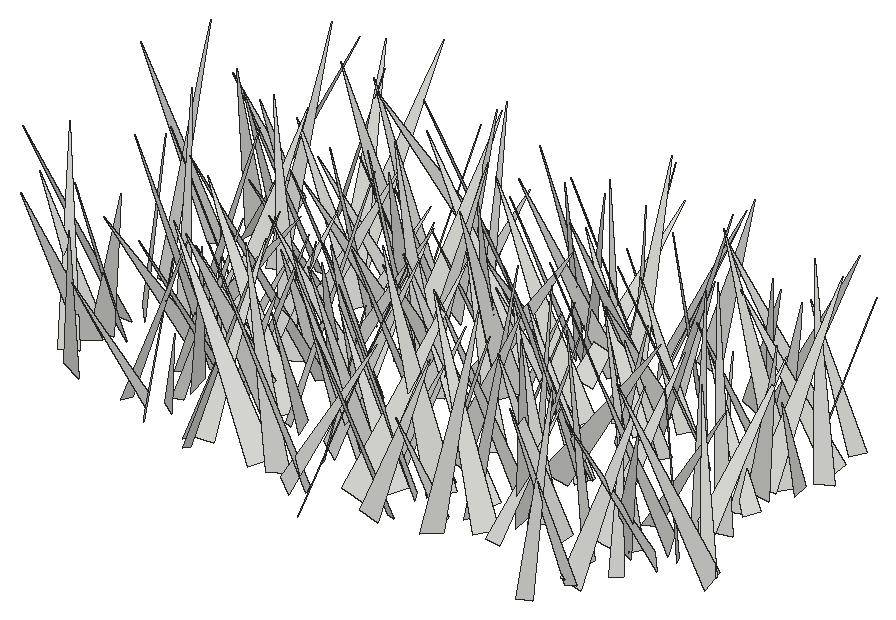
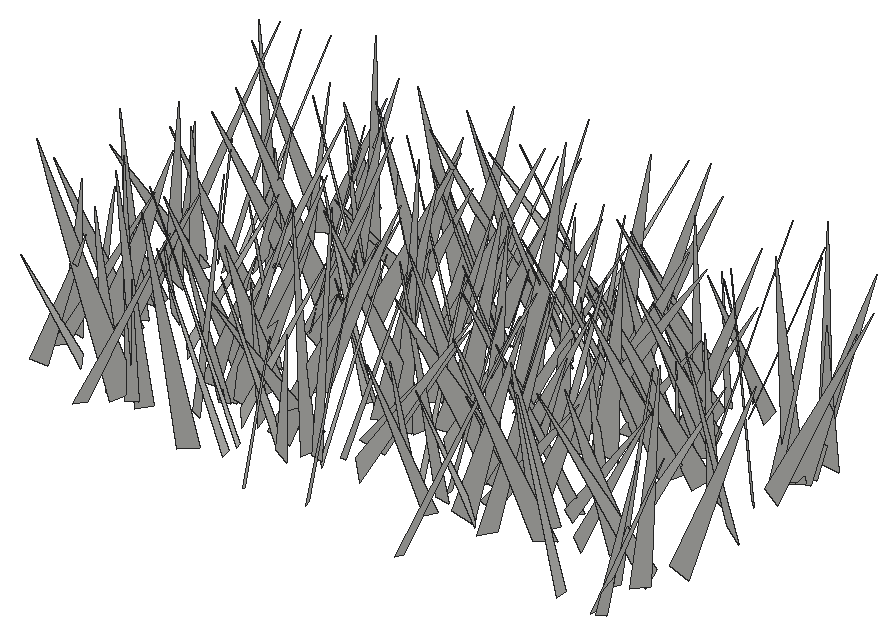
# SketchUp Ruby script. Lengths in inches.
U = 1.inch
M = Sketchup.active_model
def pt(a) = Geom::Point3d.new(a.map { |v| v * U })
def face(e, loops, mat)
  f = e.add_face(loops[0].map { |a| pt(a) })
  loops[1..].each { |l| e.add_face(l.map { |a| pt(a) }).erase! }
  f.material = f.back_material = mat if mat
  f
end
# faces: each face lists its corners as indices into pts; further lists are holes
def faces(e, pts, list, mat = nil) = list.each { |f| face(e, (f[0].is_a?(Array) ? f : [f]).map { |l| l.map { |i| pts[i] } }, mat) }
# xy, xz, yz: faces in a plane at the given z, y or x. An outline is a flat list of corners, or four numbers for a rectangle; further outlines are holes
def ring(l) = l.size == 4 ? [[l[0], l[1]], [l[2], l[1]], [l[2], l[3]], [l[0], l[3]]] : l.each_slice(2).to_a
def flat(e, list, mat, &to3) = list.each { |f| face(e, (f[0].is_a?(Array) ? f : [f]).map { |l| ring(l).map { |u, v| to3.(u, v) } }, mat) }
def xy(e, z, list, mat = nil) = flat(e, list, mat) { |x, y| [x, y, z] }
def xz(e, y, list, mat = nil) = flat(e, list, mat) { |x, z| [x, y, z] }
def yz(e, x, list, mat = nil) = flat(e, list, mat) { |y, z| [x, y, z] }
def lines(e, pts, list) = list.each { |a, b| e.add_line(pt(pts[a]), pt(pts[b])) }
# prism: a flat outline (further loops are holes) pulled along v
def prism(e, loops, v, mat = nil)
  f = face(e, loops, mat); d = Geom::Vector3d.new(v.map { |x| x * U })
  f.pushpull(f.normal.samedirection?(d) ? d.length : -d.length)
end
def box(e, o, s, mat = nil) = prism(e, [[o, [o[0] + s[0], o[1], o[2]], [o[0] + s[0], o[1] + s[1], o[2]], [o[0], o[1] + s[1], o[2]]]], [0, 0, s[2]], mat)
def at(x, y, z, deg = 0) = Geom::Transformation.translation(pt([x, y, z])) * Geom::Transformation.rotation(ORIGIN, Z_AXIS, deg.degrees)
def axes(o, x, y, z) = Geom::Transformation.new([*x, 0, *y, 0, *z, 0, *pt(o).to_a, 1])
def part(name) = M.definitions.add(name)
# library, detail: a bought-in or finely detailed component or shape, given as its bounding box
def library(name, o, s) = part(name).tap { |d| box(d.entities, o, s) }
def detail(e, o, s) = box(e.add_group.entities, o, s)
def put(e, d, t, mat = nil) = e.add_instance(d, t).tap { |i| i.material = mat if mat }
def group(e, t, mat = nil) = e.add_group.tap { |g| g.transformation = t; g.material = mat if mat }.entities
root = M.entities
c1 = part("fur_instance\#9")
p = [[0.8125,0,1.79],[0.67,-0.02,1.48],[0,-0.11,0],[0,0.11,0]]
faces(c1.entities,p,[[0,1,2,3]])
put(root,c1,axes([463.09,264.2,-21.66],[-4.74866,-3.13825,0.27488],[-2.86364,4.50737,1.98925],[1.31291,-1.51952,5.33303]))
put(root,c1,axes([483.28,262.19,-21.66],[-3.66042,-4.84933,0.70173],[-4.78346,3.34689,-1.82316],[-1.06154,1.63996,5.79575]))
put(root,c1,axes([482.21,261.42,-21.66],[1.25839,-5.65908,2.69216],[-6.0262,-0.33916,2.10388],[1.71982,2.95233,5.40207]))
put(root,c1,axes([477.375,261.69,-21.66],[-7.14593,-4.06809,0.00282],[-3.91681,6.87864,-2.22635],[-1.09909,1.93614,7.91562]))
put(root,c1,axes([476.01,261.17,-21.66],[3.46284,5.45761,0.55951],[5.19477,-3.049,-2.40992],[1.76435,-1.73432,5.99742]))
put(root,c1,axes([457.36,264.17,-21.66],[-1.15928,-6.64992,1.1524],[-6.36185,1.46707,2.06591],[2.25307,0.72087,6.42631]))
put(root,c1,axes([486.22,263.67,-21.66],[-4.22859,-0.79072,0.99748],[-0.41595,4.12901,1.5098],[1.20299,-1.35177,4.02824]))
put(root,c1,axes([495.81,259.29,-21.66],[-6.32088,1.55628,0.92222],[1.03646,5.86264,-2.78949],[1.48264,2.53644,5.88169]))
put(root,c1,axes([496.86,262.39,-21.66],[-1.92463,-5.23066,1.71698],[-5.26178,1.21283,-2.20335],[-1.6191,2.27625,5.1195]))
put(root,c1,axes([474.71,262.17,-21.66],[-1.73257,6.85044,2.42635],[7.20837,1.30251,1.46979],[-0.92468,-2.68187,6.91158]))
put(root,c1,axes([464.72,264.19,-21.66],[-1.05562,-3.90874,0.84941],[-3.49411,1.32871,1.77194],[1.94702,0.26528,3.64044]))
put(root,c1,axes([473.16,262.53,-21.66],[-5.71693,5.39586,0.3581],[5.20349,5.34707,2.50186],[-1.47216,-2.05434,7.45247]))
put(root,c1,axes([478.94,258.78,-21.66],[6.66219,5.05954,0.23915],[4.47229,-6.06129,3.64695],[-2.37798,2.77537,7.52884]))
put(root,c1,axes([486.45,262.13,-21.66],[6.53232,-2.04401,3.08815],[-2.89411,-6.72439,1.67109],[-2.31057,2.64395,6.63752]))
put(root,c1,axes([464.46,262.16,-21.66],[3.7445,3.22853,1.26331],[2.91821,-3.9391,1.41711],[-1.87174,0.31742,4.73672]))
put(root,c1,axes([468.5625,261.15,-21.66],[5.48783,2.36239,1.1528],[1.72376,-5.24883,2.55038],[-1.98455,1.97355,5.40302]))
put(root,c1,axes([496.82,262.46,-21.66],[0.16958,6.97336,1.46095],[6.91324,0.19239,-1.72074],[1.72314,-1.45812,6.75984]))
put(root,c1,axes([479.39,265.73,-21.66],[-7.48109,-1.28394,1.71532],[-0.94889,7.57103,1.5286],[1.92105,-1.26035,7.43496]))
put(root,c1,axes([499.0625,267.78,-21.66],[-5.37416,-4.85351,0.14678],[-4.51514,5.07548,2.5125],[1.7865,-1.77274,6.79157]))
put(root,c1,axes([482.9375,265.05,-21.66],[-5.86461,-3.9483,0.52207],[-3.9663,5.70596,-1.40208],[-0.36068,1.452,6.92942]))
put(root,c1,axes([496.57,267.59,-21.66],[-0.05965,-7.49908,0.31223],[-6.76708,0.1888,3.24163],[3.24657,0.25574,6.76251]))
put(root,c1,axes([493.22,266.27,-21.66],[-6.6748,0.96554,1.83268],[1.43583,6.61336,1.7452],[1.49311,-2.0433,6.51456]))
put(root,c1,axes([489.83,266.86,-21.66],[7.80174,-0.94154,1.76979],[-0.49694,-7.7978,-1.95786],[-1.94209,-1.78708,7.61055]))
put(root,c1,axes([469.38,268.36,-21.66],[6.1806,-4.85252,1.92283],[-3.89661,-6.27237,-3.30423],[-3.47285,-1.59827,7.12944]))
put(root,c1,axes([468.61,262.53,-21.66],[-3.2571,5.60614,0.8435],[5.30317,3.35677,-1.83235],[2.00417,0.22864,6.21933]))
put(root,c1,axes([462.03,263.6,-21.66],[5.46763,0.70402,1.09334],[0.38726,-5.3924,1.5356],[-1.2414,1.41859,5.29457]))
put(root,c1,axes([455.94,267.78,-21.66],[2.22572,-6.24997,0.53761],[-6.03536,-2.28904,-1.62473],[-1.71046,-0.05581,6.43243]))
put(root,c1,axes([481.73,264.88,-21.66],[-4.33384,4.15795,0.46311],[4.09626,4.08164,1.68703],[-0.85069,-1.52868,5.76409]))
put(root,c1,axes([472.49,267.375,-21.66],[5.01646,-0.03484,2.02413],[0.79085,-4.94522,-2.0451],[-1.86357,-2.19241,4.58078]))
put(root,c1,axes([467.9,262.12,-21.66],[7.02675,2.35333,1.41841],[1.60681,-6.67867,3.12071],[-2.22895,2.60433,6.72121]))
put(root,c1,axes([488.88,264.25,-21.66],[-3.57557,6.64036,0.56629],[6.42877,3.26724,2.27945],[-1.75672,-1.55901,7.1891]))
put(root,c1,axes([464.4,267.42,-21.66],[6.47505,-0.26988,1.20187],[0.07267,-6.33614,-1.81428],[-1.22965,-1.79557,6.22153]))
put(root,c1,axes([503.21,267.97,-21.66],[-7.55604,-1.18176,1.01335],[-0.88861,7.39753,2.00103],[1.27821,-1.84315,7.38147]))
put(root,c1,axes([479.98,262.75,-21.66],[0.04279,8.23701,0.26485],[7.98617,0.02394,-2.03491],[2.0346,-0.26721,7.98181]))
put(root,c1,axes([484.01,266.13,-21.66],[-5.61004,5.72169,2.32507],[6.16954,5.3361,1.75473],[0.28367,-2.89906,7.81865]))
put(root,c1,axes([496.12,265.1,-21.66],[-7.03444,-1.19576,1.59787],[-1.52444,6.99776,-1.47438],[1.28808,1.75153,6.98136]))
put(root,c1,axes([490.02,263.52,-21.66],[-3.33289,3.23483,0.32122],[2.5841,2.91556,-2.549],[1.97223,1.64647,3.88264]))
put(root,c1,axes([478.18,266.27,-21.66],[-1.48445,-5.73193,2.26963],[-5.6541,0.33538,-2.85107],[-2.45713,2.69116,5.18942]))
put(root,c1,axes([479.74,266.53,-21.66],[2.31497,4.33574,1.17317],[4.28428,-1.73503,-2.04175],[1.34907,-1.93005,4.47091]))
put(root,c1,axes([498.38,264.85,-21.66],[-4.64664,1.60589,0.29185],[1.45378,4.47236,-1.46283],[0.74202,1.29401,4.69365]))
put(root,c1,axes([460.67,271.62,-21.66],[-6.33754,-5.19611,0.8236],[-4.02771,5.62162,4.47406],[3.3846,-3.03975,6.86635]))
put(root,c1,axes([498.58,269.875,-21.66],[-6.83559,-3.49227,1.59422],[-2.83471,6.78714,2.71329],[2.5888,-1.7893,7.18049]))
put(root,c1,axes([456.85,269.5625,-21.66],[-3.15588,-6.30761,0.73503],[-6.08642,3.23856,1.65924],[1.81157,-0.10755,6.85511]))
put(root,c1,axes([467.08,267.49,-21.66],[3.19208,-3.97574,0.46961],[-3.91795,-2.97897,1.41133],[0.82265,1.2392,4.89939]))
put(root,c1,axes([483.3,267.73,-21.66],[-3.35024,-7.10363,1.41562],[-6.97339,2.74138,-2.74705],[-1.95891,2.39017,7.35795]))
put(root,c1,axes([475.38,266.2,-21.66],[3.97232,6.71602,1.21655],[6.692,-3.55551,-2.22255],[1.34242,-2.14887,7.47961]))
put(root,c1,axes([487.2,266.84,-21.66],[-4.10469,4.34568,0.4298],[4.19686,3.76273,2.03626],[-1.20665,-1.6956,5.62024]))
put(root,c1,axes([480.36,266.53,-21.66],[3.62784,4.7769,0.79864],[4.78599,-3.38301,-1.50576],[0.74217,-1.53438,5.80626]))
put(root,c1,axes([482.87,267.64,-21.66],[5.29628,3.42643,1.15131],[3.61426,-4.98862,-1.7797],[0.0553,-2.11891,6.05175]))
put(root,c1,axes([455.875,268.94,-21.66],[2.61473,-6.42495,0.46001],[-6.33227,-2.47287,1.45453],[1.18065,0.96609,6.78241]))
put(root,c1,axes([476.03,264.82,-21.66],[3.78632,3.0497,0.88341],[2.42458,-3.66486,2.25998],[-2.05,1.29824,4.30457]))
put(root,c1,axes([487.13,265.07,-21.66],[-7.34355,0.30763,3.29021],[-0.75169,7.65215,-2.39318],[3.21793,2.48952,6.94946]))
put(root,c1,axes([464.78,269.43,-21.66],[-1.76635,-5.02439,0.02248],[-4.81779,1.68692,-1.51928],[-1.42615,0.52421,5.10454]))
put(root,c1,axes([491.2,267.39,-21.66],[-2.35431,6.5098,1.98677],[6.74258,1.94391,1.62058],[-0.92858,-2.38982,6.73008]))
put(root,c1,axes([455.63,268.67,-21.66],[-4.26864,3.3889,1.68719],[3.78174,3.93314,1.66776],[0.17248,-2.36607,5.18889]))
put(root,c1,axes([455.63,266.04,-21.66],[-1.06159,6.87885,0.56166],[6.76624,0.92524,1.45707],[-1.36093,-0.76575,6.80607]))
put(root,c1,axes([474.82,271.05,-21.66],[5.51708,-5.76072,0.82028],[-5.55442,-5.55067,-1.6234],[-1.73412,-0.54876,7.80952]))
put(root,c1,axes([464.41,265.49,-21.66],[5.42,0.95377,1.93695],[-0.10115,-5.11614,2.80228],[-2.15667,2.63692,4.73638]))
put(root,c1,axes([473.36,269.98,-21.66],[-6.08575,-1.31512,1.93305],[-0.80976,6.24223,1.69745],[2.19329,-1.34444,5.99037]))
put(root,c1,axes([488.09,268.9,-21.66],[-2.1287,-6.56011,1.58213],[-6.38568,1.42177,-2.69649],[-2.18201,2.23898,6.34786]))
put(root,c1,axes([482.17,269.72,-21.66],[1.4912,-7.63112,1.5604],[-7.07021,-0.65953,3.53123],[3.26816,2.05513,6.92734]))
put(root,c1,axes([490.82,266.37,-21.66],[3.07038,6.62387,1.59445],[6.28566,-3.42873,2.13997],[-2.62838,-0.46188,6.98022]))
put(root,c1,axes([470.73,268.14,-21.66],[-4.85114,5.94494,0.47809],[5.69058,4.42924,2.66526],[-1.78556,-2.03568,7.19529]))
put(root,c1,axes([464.12,269.57,-21.66],[1.30343,6.50873,4.51627],[7.0846,-3.00591,2.28737],[-3.54523,-3.61388,6.23141]))
put(root,c1,axes([487.41,269.79,-21.66],[6.19787,3.91116,1.13836],[4.069,-5.84754,-2.06304],[0.19042,-2.34857,7.0324]))
put(root,c1,axes([455.95,271.08,-21.66],[-2.71774,-6.73125,0.47193],[-6.54696,2.5072,-1.9416],[-1.63394,1.15011,6.99472]))
put(root,c1,axes([468.02,266.79,-21.66],[5.42222,1.22065,1.50489],[0.3801,-5.05507,2.73075],[-1.90005,2.47215,4.84081]))
put(root,c1,axes([495.1,267.53,-21.66],[-1.51128,6.4389,0.97646],[6.11666,1.74753,-2.05657],[2.23592,-0.42848,6.28601]))
put(root,c1,axes([500.01,268.71,-21.66],[-4.46035,-2.40279,1.6408],[-2.85913,4.17643,-1.65628],[0.53948,2.26814,4.788]))
put(root,c1,axes([502.68,268.27,-21.66],[-0.8171,5.77252,0.59098],[5.63961,0.64951,1.4532],[-1.36602,-0.77139,5.64605]))
put(root,c1,axes([497.35,268.07,-21.66],[-7.36083,-0.13148,0.37404],[-0.23398,7.05478,-2.12469],[0.32007,2.13349,7.04874]))
put(root,c1,axes([490.09,272.2,-21.66],[-5.41835,-3.58553,1.38238],[-3.2455,5.54933,1.6725],[2.0576,-0.68883,6.27832]))
put(root,c1,axes([467.46,270.59,-21.66],[-3.75948,2.94392,0.27379],[2.73653,3.29698,2.12525],[-1.1194,-1.82718,4.27594]))
put(root,c1,axes([461.97,269.82,-21.66],[0.15011,3.96157,1.30257],[3.86973,0.35348,-1.52101],[1.55431,-1.26265,3.66102]))
put(root,c1,axes([474.12,272.7,-21.66],[-5.52668,-3.91053,1.22579],[-3.5737,5.60606,1.77193],[2.00587,-0.78663,6.53427]))
put(root,c1,axes([470.54,273.08,-21.66],[0.16634,-6.6201,0.01552],[-6.42128,-0.15757,1.61124],[1.61035,0.05552,6.42319]))
put(root,c1,axes([474.13,272.2,-21.66],[-7.00038,0.48524,0.02911],[0.47648,6.76613,1.79834],[-0.09628,-1.796,6.78283]))
put(root,c1,axes([471.55,267.09,-21.66],[5.15692,6.28398,0.1894],[5.87834,-4.90651,2.73667],[-2.22922,1.59869,7.6546]))
put(root,c1,axes([487.97,271.95,-21.66],[4.31656,-7.06636,0.27005],[-6.24466,-3.6606,4.0303],[3.31821,2.3034,7.23345]))
put(root,c1,axes([463.9,269.98,-21.66],[1.76698,3.75792,1.11012],[3.4505,-2.06932,1.51278],[-1.85698,-0.26926,3.86726]))
put(root,c1,axes([496.09,271.05,-21.66],[4.90095,-2.69617,0.00541],[-2.57457,-4.67657,1.67032],[0.80058,1.46597,5.33842]))
put(root,c1,axes([456.32,272.35,-21.66],[5.45903,4.38742,2.52703],[5.0114,-5.21201,-1.77686],[-0.72192,-3.00365,6.77446]))
put(root,c1,axes([469.76,272.59,-21.66],[-3.41379,-7.32141,0.63154],[-6.65452,2.7845,-3.69049],[-3.11756,2.07349,7.18591]))
put(root,c1,axes([489.42,273.13,-21.66],[-2.75065,-6.97463,1.22589],[-6.99898,2.47729,-1.60986],[-1.07823,1.71227,7.32256]))
put(root,c1,axes([462.47,268.2,-21.66],[-6.96158,0.42843,3.50828],[-1.43896,6.73486,-3.67782],[3.22816,3.92599,5.92628]))
put(root,c1,axes([468.37,274.08,-21.66],[3.73723,-3.51523,0.8829],[-3.22394,-3.80362,-1.49732],[-1.65607,-0.52811,4.90732]))
put(root,c1,axes([466.13,270.51,-21.66],[1.18506,6.07091,0.5983],[5.8889,-0.9794,-1.72625],[1.5921,-0.89616,5.93973]))
put(root,c1,axes([494.11,273.41,-21.66],[-5.74525,-5.95088,0.61636],[-5.93253,5.55629,-1.65334],[-0.77329,1.58601,8.10478]))
put(root,c1,axes([460.12,272.41,-21.66],[4.62991,-4.98565,0.093],[-4.3743,-3.99984,3.34189],[2.39393,2.33366,5.92659]))
put(root,c1,axes([463.6,271.98,-21.66],[3.57113,-2.0967,0.79041],[-2.23153,-3.1932,1.61171],[0.20288,1.78359,3.81464]))
put(root,c1,axes([489.68,272.76,-21.66],[-3.57331,4.48467,0.98446],[4.4978,3.16833,1.89248],[-0.92266,-1.92337,5.41289]))
put(root,c1,axes([478.97,274.625,-21.66],[5.01755,-2.86523,2.69296],[-2.1597,-5.65647,-1.99435],[-3.28592,-0.6574,5.42291]))
put(root,c1,axes([476.15,276.95,-21.66],[4.64507,-4.79979,0.2726],[-4.36308,-4.36804,-2.56373],[-2.01887,-1.6035,6.16782]))
put(root,c1,axes([465.91,274.79,-21.66],[5.21952,0.68023,0.61562],[0.83808,-4.98198,-1.60081],[-0.37326,-1.674,5.01433]))
put(root,c1,axes([499.94,270.75,-21.66],[-7.67594,0.43258,1.18162],[-0.05572,7.18028,-2.99063],[1.25708,2.9597,7.0826]))
put(root,c1,axes([483.38,272.32,-21.66],[-1.50811,5.89701,0.63499],[5.61901,1.21081,2.10069],[-1.89858,-1.1007,5.71281]))
put(root,c1,axes([499.87,270.71,-21.66],[-2.9172,5.75801,0.16061],[5.28877,2.74872,-2.48273],[2.2824,0.99014,5.95825]))
put(root,c1,axes([487.06,275.74,-21.66],[-5.99784,0.36822,0.31916],[0.44096,5.77868,1.61988],[0.20737,-1.63795,5.78668]))
put(root,c1,axes([500.14,272.85,-21.66],[0.70044,7.59304,1.85976],[7.56257,-1.13109,1.76971],[-1.98005,-1.63401,7.41708]))
put(root,c1,axes([466.85,273.35,-21.66],[-1.50956,7.97784,1.83345],[8.07703,1.14872,1.65178],[-1.3301,-2.07864,7.94961]))
put(root,c1,axes([458.59,273.23,-21.66],[1.63726,6.8228,1.57078],[6.72877,-1.9791,1.58281],[-1.9343,-1.10957,6.83563]))
put(root,c1,axes([481.88,277.03,-21.66],[6.81977,1.54998,0.06465],[1.44583,-6.24479,-2.79788],[0.56233,-2.74155,6.40965]))
put(root,c1,axes([472.35,272.96,-21.66],[-2.22642,5.28944,0.76409],[4.89566,2.35054,-2.00661],[2.14349,0.12554,5.37668]))
put(root,c1,axes([476.19,275.09,-21.66],[-0.9931,7.68396,2.84346],[8.04191,0.36629,1.81887],[-1.56723,-2.98953,7.53135]))
put(root,c1,axes([479.78,278.17,-21.66],[5.20163,-5.29224,1.8402],[-4.95757,-5.51713,-1.85336],[-2.61089,-0.0677,7.18539]))
put(root,c1,axes([461.92,272.91,-21.66],[-4.61251,5.93847,1.25396],[5.3205,4.71401,-2.75381],[2.92064,0.79104,6.99694]))
put(root,c1,axes([478.12,278.53,-21.66],[-1.25565,-8.18969,1.33935],[-8.04493,1.53362,1.83538],[2.03567,1.00923,8.07955]))
put(root,c1,axes([461.29,275.84,-21.66],[-4.82792,-3.85999,0.34861],[-3.62589,4.30173,-2.58417],[-1.36894,2.21934,5.6152]))
put(root,c1,axes([468.7,276.99,-21.66],[4.45492,4.83666,0.95124],[4.56601,-3.56591,-3.25273],[1.85733,-2.83468,5.71483]))
put(root,c1,axes([488.74,277.09,-21.66],[3.06956,3.90435,1.71137],[4.25532,-2.68017,-1.51785],[0.25498,-2.27325,4.72887]))
put(root,c1,axes([499.9,275.875,-21.66],[-3.00277,4.1066,0.06153],[3.92812,2.84936,1.52829],[-1.19912,-0.94951,4.85234]))
put(root,c1,axes([498.86,277.8125,-21.66],[1.26894,-6.32164,1.3833],[-6.3592,-0.957,1.46001],[1.19887,1.6149,6.28026]))
put(root,c1,axes([474.04,276.36,-21.66],[-6.46812,-3.13785,1.21731],[-3.3431,6.29489,-1.53709],[0.38946,1.92167,7.02282]))
put(root,c1,axes([466.18,279.95,-21.66],[-2.99336,-6.46525,0.18966],[-6.30073,2.9619,1.52434],[1.46161,-0.47255,6.9596]))
put(root,c1,axes([499.04,275.34,-21.66],[-3.77654,1.99621,0.89861],[1.50689,3.67022,-1.82025],[1.58796,1.26459,3.86442]))
put(root,c1,axes([477.2,277.54,-21.66],[3.63581,-6.29578,1.08718],[-5.74464,-2.67402,3.72648],[2.79605,2.69271,6.24254]))
put(root,c1,axes([480.76,277.59,-21.66],[2.90459,3.11145,0.76807],[3.13189,-2.53582,-1.57117],[0.67994,-1.61126,3.9559]))
put(root,c1,axes([470.27,280.4,-21.66],[7.22069,-3.00234,1.05262],[-2.62839,-7.10035,-2.22196],[-1.79266,-1.6827,7.49769]))
put(root,c1,axes([491.67,277.95,-21.66],[-1.39517,3.65073,1.37856],[3.73252,0.82124,1.60268],[-1.13865,-1.78115,3.56451]))
put(root,c1,axes([485.2,278.04,-21.66],[-7.15301,3.97515,0.71331],[4.02795,6.91641,1.848],[-0.2937,-1.95899,7.97197]))
put(root,c1,axes([469.38,280.47,-21.66],[1.60402,-6.13136,0.73735],[-5.58582,-1.76536,-2.52831],[-2.63361,0.00991,5.81155]))
put(root,c1,axes([497.26,276.23,-21.66],[1.37607,4.21587,0.41156],[3.82506,-1.42264,1.78368],[-1.81985,0.19763,4.06025]))
put(root,c1,axes([494.35,278.78,-21.66],[-5.23491,-4.53939,0.15815],[-4.43832,5.06084,-1.65066],[-0.96564,1.34804,6.72946]))
put(root,c1,axes([474.78,278.55,-21.66],[-4.9499,-5.12629,0.49866],[-4.98162,4.58947,-2.26921],[-1.30806,1.92014,6.75508]))
put(root,c1,axes([474.51,276.19,-21.66],[6.67924,-1.26552,2.75336],[-2.18749,-6.62541,2.26131],[-2.097,2.88046,6.41095]))
put(root,c1,axes([500.49,279.78,-21.66],[4.01864,-1.00258,0.99057],[-0.63294,-3.95809,-1.43832],[-1.25928,-1.21004,3.88405]))
put(root,c1,axes([498.57,279.72,-21.66],[-1.67937,-5.43767,0.87836],[-5.25266,1.30456,-1.96667],[-1.65811,1.37475,5.34049]))
put(root,c1,axes([454.89,276.06,-21.66],[3.59561,7.30217,1.1805],[7.09033,-3.77639,1.76345],[-2.10771,-0.24675,7.94609]))
put(root,c1,axes([488.53,282.13,-21.66],[5.3138,-2.81187,1.14067],[-1.98861,-4.96443,-2.9739],[-2.29198,-2.2118,5.22484]))
put(root,c1,axes([488.16,281.79,-21.66],[-0.28332,-7.79704,0.77926],[-7.68212,0.12267,-1.56569],[-1.54472,0.82004,7.64347]))
put(root,c1,axes([463.92,280.4,-21.66],[-1.49578,-4.28811,0.26565],[-3.87905,1.22698,-2.03551],[-1.84701,0.89578,4.0598]))
put(root,c1,axes([478.81,283.33,-21.66],[-5.2943,-3.28141,1.0592],[-2.29433,4.80125,3.40634],[2.57403,-2.46971,5.21479]))
put(root,c1,axes([472.74,283.71,-21.66],[-3.72735,-5.65721,0.3773],[-4.71825,3.34531,3.54775],[3.14396,-1.68653,5.77153]))
put(root,c1,axes([467.91,279.64,-21.66],[-2.85535,-4.62994,1.75531],[-4.89429,2.33192,-1.81068],[-0.75056,2.40755,5.12941]))
put(root,c1,axes([488.83,279.47,-21.66],[-4.99082,4.3261,0.4502],[4.29852,4.80129,1.51542],[-0.66378,-1.43477,6.4286]))
put(root,c1,axes([499.73,279.52,-21.66],[-2.9065,7.574,1.65107],[7.44857,2.24028,2.83534],[-2.14716,-2.4809,7.60092]))
put(root,c1,axes([471.26,282.61,-21.66],[-5.10979,-2.8974,1.28802],[-2.4355,5.15064,1.92434],[2.03034,-1.11347,5.54994]))
put(root,c1,axes([463.72,279.8,-21.66],[1.55014,5.60518,1.20615],[5.3228,-0.94254,-2.46072],[2.13086,-1.72318,5.26933]))
put(root,c1,axes([466.02,281.0625,-21.66],[-3.70212,4.89762,1.86065],[5.19102,3.12087,2.11373],[-0.70854,-2.72541,5.76407]))
put(root,c1,axes([454.44,281.71,-21.66],[-0.79345,-6.87819,1.77521],[-6.83318,0.25089,-2.08208],[-1.94125,1.92821,6.60333]))
put(root,c1,axes([490.68,281.18,-21.66],[-3.29735,3.76242,1.32483],[3.9802,2.99017,1.41439],[-0.2628,-1.92005,4.79874]))
put(root,c1,axes([498.5625,278.76,-21.66],[-1.75958,6.89289,0.89816],[6.66639,1.93582,-1.79628],[1.96924,-0.39424,6.88342]))
put(root,c1,axes([472.59,277.15,-21.66],[-6.00676,5.62271,0.83771],[4.81686,5.68135,-3.59416],[3.01902,2.12255,7.40122]))
put(root,c1,axes([490.35,278.5,-21.66],[7.12647,2.20024,1.82821],[1.44023,-6.99989,2.8102],[-2.47167,2.26505,6.90872]))
put(root,c1,axes([500.64,283.07,-21.66],[-6.49837,1.01991,0.13564],[1.01971,6.26851,1.71854],[-0.13717,-1.71841,6.34946]))
put(root,c1,axes([483.36,283.8125,-21.66],[0.24896,-7.3468,1.55373],[-6.97419,-0.80255,-2.67734],[-2.78393,1.35351,6.84612]))
put(root,c1,axes([468.35,282.57,-21.66],[-2.5232,4.5633,1.53247],[4.25008,1.29942,3.12842],[-2.26029,-2.65076,4.17172]))
put(root,c1,axes([466.23,281.25,-21.66],[1.55212,3.88569,0.28277],[3.69063,-1.36892,-1.44671],[1.24813,-0.78428,3.92616]))
put(root,c1,axes([479.39,284.68,-21.66],[-5.06426,-4.56399,0.84014],[-4.29824,5.08189,1.69768],[1.74956,-0.72593,6.60262]))
put(root,c1,axes([478.31,281.14,-21.66],[-3.77529,6.85051,0.02559],[5.94676,3.26269,3.89536],[-3.40091,-1.89957,6.78296]))
put(root,c1,axes([480.08,284.27,-21.66],[-3.33298,-6.74445,1.96036],[-6.484,3.7887,2.01069],[2.69971,0.77298,7.24938]))
put(root,c1,axes([461.41,282.74,-21.66],[-3.32714,-4.87132,0.7615],[-4.7527,2.92423,-2.05917],[-1.31203,1.7603,5.52806]))
put(root,c1,axes([489.04,284.56,-21.66],[-3.9717,-6.10655,1.7462],[-5.81347,4.32471,1.90107],[2.55787,0.34722,7.03209]))
put(root,c1,axes([488.62,282.375,-21.66],[-0.11529,-4.79427,2.44231],[-5.06003,0.9271,1.58106],[1.8292,2.26244,4.52754]))
put(root,c1,axes([480.81,284.14,-21.66],[7.66875,0.29762,1.40281],[0.64374,-7.5341,-1.92071],[-1.28143,-2.00373,7.43029]))
put(root,c1,axes([455.2,284.5,-21.66],[6.33398,-2.31725,1.64534],[-1.9481,-6.46653,-1.60778],[-2.06922,-1.00519,6.55011]))
put(root,c1,axes([456.36,285.1875,-21.66],[6.05103,1.03829,2.78411],[2.19851,-5.8136,-2.61017],[-1.99898,-3.2509,5.55698]))
put(root,c1,axes([501.05,281.33,-21.66],[-0.8728,6.82324,1.17968],[6.78553,0.6058,1.51645],[-1.38016,-1.33658,6.7096]))
put(root,c1,axes([486.65,283.24,-21.66],[-5.69424,-4.56861,0.52497],[-4.47673,5.31586,-2.29625],[-1.05201,2.10752,6.92992]))
put(root,c1,axes([493.01,285.75,-21.66],[-1.64763,-7.14584,1.34901],[-6.49832,2.06763,3.01567],[3.26416,0.50931,6.68457]))
put(root,c1,axes([466.42,285.07,-21.66],[-7.9399,0.37328,2.34081],[0.92834,8.01881,1.87016],[2.18103,-2.05426,7.72553]))
put(root,c1,axes([487.23,279.61,-21.66],[-7.03666,4.34174,0.35439],[3.96979,6.66848,-2.87454],[1.79361,2.2741,7.75256]))
put(root,c1,axes([491.99,285.82,-21.66],[0.44147,-7.17503,0.62576],[-6.54369,-0.13768,3.03788],[3.00878,0.75334,6.51516]))
put(root,c1,axes([471.04,283.57,-21.66],[-2.12698,-6.60371,3.80122],[-7.1046,3.14508,1.48842],[2.75369,3.0136,6.77625]))
put(root,c1,axes([477.26,283.86,-21.66],[-5.76145,-5.93812,0.42997],[-5.44241,5.01036,-3.73055],[-2.41379,2.87671,7.38502]))
put(root,c1,axes([468.77,284.48,-21.66],[-0.03383,-6.90938,2.82252],[-7.12958,-0.80509,-2.05628],[-2.20801,2.70547,6.5964]))
put(root,c1,axes([485.42,282.73,-21.66],[-5.55203,-0.57439,2.02149],[-1.15794,5.60149,-1.58866],[1.75372,1.88009,5.3508]))
put(root,c1,axes([494.51,285.47,-21.66],[1.53942,-5.44162,0.89342],[-5.38829,-1.28703,1.44538],[1.17292,1.22946,5.46735]))
put(root,c1,axes([459.17,281.43,-21.66],[-6.96616,2.88196,1.8212],[2.05018,6.85162,-3.00033],[2.72382,2.21349,6.91601]))
put(root,c1,axes([493.77,285.56,-21.66],[6.6749,-4.96789,0.00129],[-4.8195,-6.47499,2.02019],[1.20515,1.62135,8.07174]))
put(root,c1,axes([463.91,282.54,-21.66],[-5.45003,5.37343,0.92209],[5.18096,5.51046,-1.48977],[1.69756,0.43353,7.50714]))
put(root,c1,axes([482.04,282.03,-21.66],[-1.93127,6.17376,0.09606],[5.65668,1.80943,-2.5656],[2.47519,0.68189,5.93825]))
put(root,c1,axes([500.32,285.49,-21.66],[-2.9134,4.03937,1.46912],[4.26943,2.51447,1.5531],[-0.49677,-2.07934,4.73205]))
put(root,c1,axes([484.7,286,-21.66],[7.11507,4.33314,0.48127],[4.20256,-6.57141,-2.9643],[1.16029,-2.76992,7.78545]))
put(root,c1,axes([470.51,285.31,-21.66],[0.36945,4.73641,1.83647],[4.53767,0.52011,-2.25427],[2.28381,-1.79961,4.18191]))
put(root,c1,axes([455.34,283.28,-21.66],[7.33228,1.89466,0.16833],[1.78282,-7.07911,2.02191],[-0.66303,1.91751,7.29821]))
put(root,c1,axes([477.05,288.92,-21.66],[-6.01376,-4.74049,2.00405],[-3.98095,6.23797,2.80955],[3.26197,-1.12665,7.12348]))
put(root,c1,axes([473.85,282.875,-21.66],[2.20032,6.76237,0.49836],[6.15454,-2.21163,2.83722],[-2.84601,0.44546,6.52083]))
put(root,c1,axes([463.13,283.64,-21.66],[-0.97355,8.05143,1.14446],[7.84551,1.23329,-2.00251],[2.14086,-0.85824,7.85896]))
put(root,c1,axes([498.41,283.79,-21.66],[4.22042,3.02936,0.44277],[2.70703,-4.0447,1.87014],[-1.43005,1.2839,4.84681]))
put(root,c1,axes([495.32,287.79,-21.66],[-6.50951,0.22142,0.60358],[0.38251,6.26967,1.82536],[0.51674,-1.85181,6.25226]))
put(root,c1,axes([483.3,283.9,-21.66],[5.52585,4.05046,1.31825],[3.69086,-5.63091,1.83015],[-2.12639,0.75214,6.60241]))
put(root,c1,axes([468.01,284.21,-21.66],[4.5765,3.32185,0.66717],[3.07667,-4.544,1.52],[-1.41913,0.86116,5.4469]))
put(root,c1,axes([468.84,290.46,-21.66],[-7.67561,-3.02253,0.64542],[-2.50236,7.09168,3.4516],[1.81396,-3.00659,7.49247]))
put(root,c1,axes([454.91,288.58,-21.66],[-4.32761,-0.50237,2.11035],[0.41917,4.42689,1.9134],[2.12844,-1.89326,3.91401]))
put(root,c1,axes([481.89,285.38,-21.66],[1.02305,5.31057,1.33507],[5.15193,-1.39366,1.59576],[-1.8553,-0.94167,5.16743]))
put(root,c1,axes([455.43,288.46,-21.66],[-5.22696,-1.19875,0.73288],[-0.94186,5.08442,1.59898],[1.04259,-1.41663,5.11873]))
put(root,c1,axes([484.66,287.2,-21.66],[6.0574,2.72005,0.2303],[2.69232,-5.86042,-1.5971],[0.45071,-1.54939,6.44516]))
put(root,c1,axes([458.29,288.12,-21.66],[6.75177,1.95337,0.7466],[2.07523,-6.56983,-1.57805],[-0.25785,-1.72661,6.84922]))
put(root,c1,axes([486.82,288.08,-21.66],[1.53835,-7.01276,2.03333],[-7.04829,-0.88366,2.28484],[1.90652,2.39168,6.80623]))
put(root,c1,axes([481.24,289.77,-21.66],[-2.96228,-3.48582,0.87467],[-2.85625,2.97145,2.16874],[2.18125,-0.843,4.02773]))
